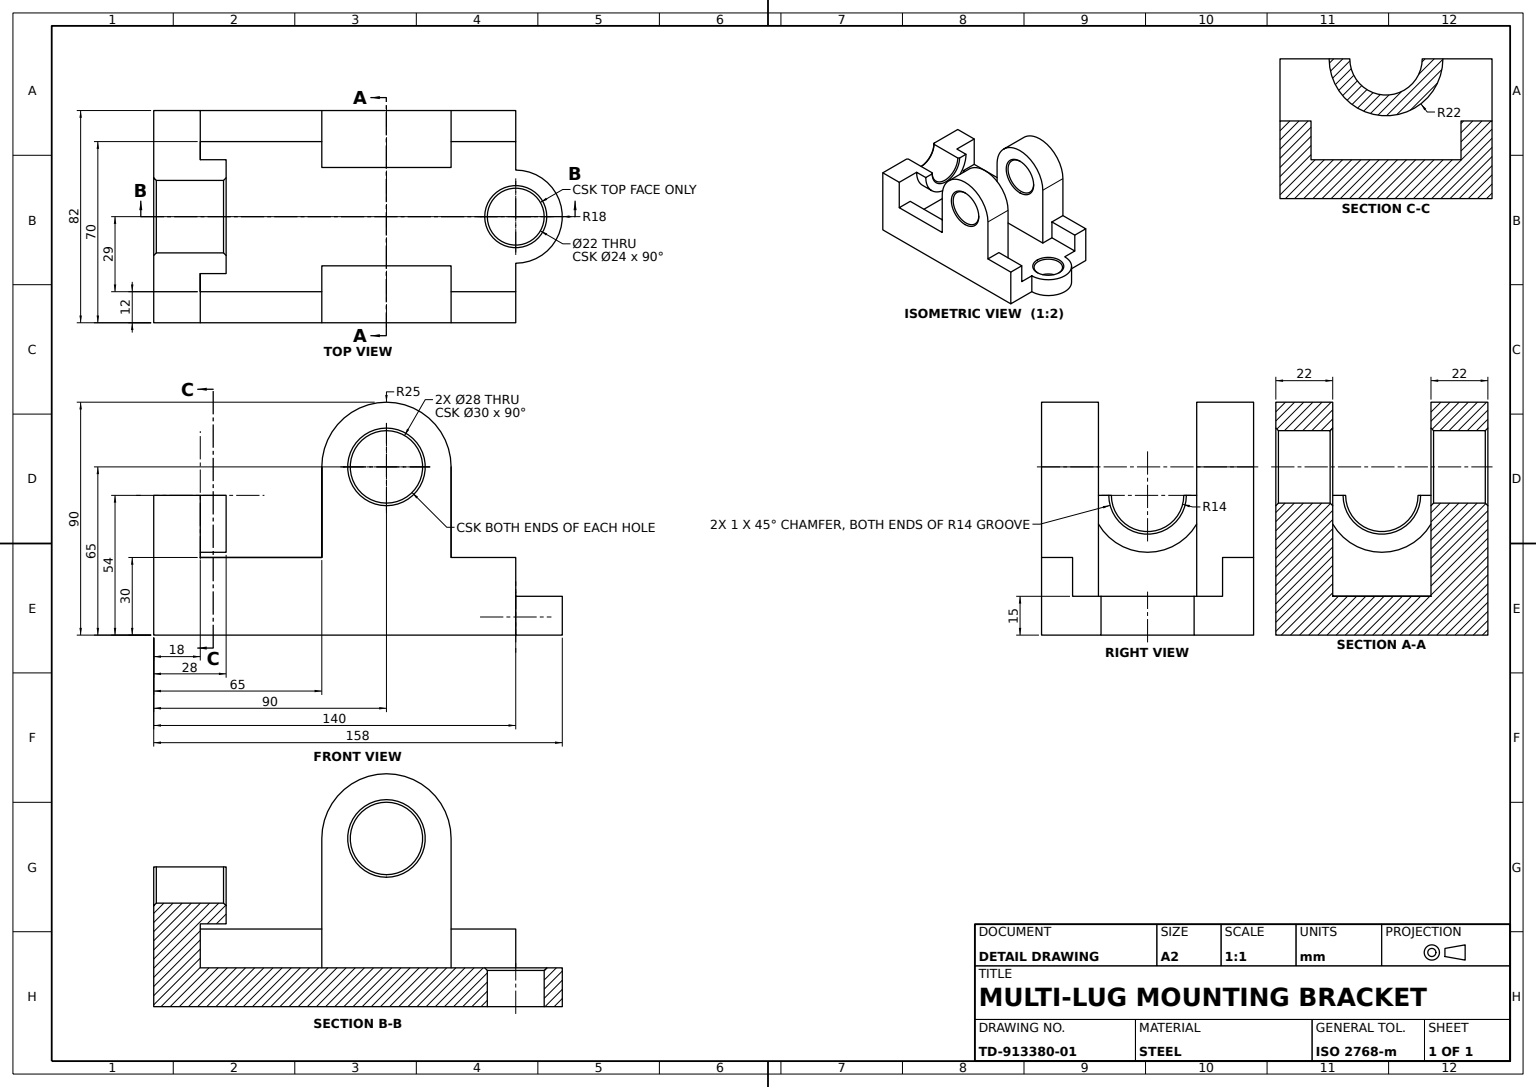
ISO-10303-21;
HEADER;
FILE_DESCRIPTION((''),'2;1');
FILE_NAME('','',(''),(''),'','','');
FILE_SCHEMA(('AUTOMOTIVE_DESIGN'));
ENDSEC;
DATA;
#1=APPLICATION_CONTEXT('');
#2=PRODUCT_CONTEXT('',#1,'mechanical');
#3=PRODUCT('','','',(#2));
#4=PRODUCT_DEFINITION_FORMATION('','',#3);
#5=PRODUCT_DEFINITION_CONTEXT('',#1,'design');
#6=PRODUCT_DEFINITION('','',#4,#5);
#7=PRODUCT_DEFINITION_SHAPE('','',#6);
#8=(LENGTH_UNIT()NAMED_UNIT(*)SI_UNIT(.MILLI.,.METRE.));
#9=(NAMED_UNIT(*)PLANE_ANGLE_UNIT()SI_UNIT($,.RADIAN.));
#10=(NAMED_UNIT(*)SI_UNIT($,.STERADIAN.)SOLID_ANGLE_UNIT());
#11=UNCERTAINTY_MEASURE_WITH_UNIT(LENGTH_MEASURE(0.005),#8,'distance_accuracy_value','');
#12=(GEOMETRIC_REPRESENTATION_CONTEXT(3)GLOBAL_UNCERTAINTY_ASSIGNED_CONTEXT((#11))GLOBAL_UNIT_ASSIGNED_CONTEXT((#8,#9,#10))REPRESENTATION_CONTEXT('',''));
#13=CARTESIAN_POINT('',(-42.,15.,54.));
#14=VERTEX_POINT('',#13);
#15=CARTESIAN_POINT('',(-42.,-15.,54.));
#16=VERTEX_POINT('',#15);
#17=CARTESIAN_POINT('',(-42.,0.,54.));
#18=DIRECTION('',(1.,0.,0.));
#19=DIRECTION('',(0.,0.,-1.));
#20=AXIS2_PLACEMENT_3D('',#17,#18,#19);
#21=CIRCLE('',#20,15.);
#22=EDGE_CURVE('',#14,#16,#21,.F.);
#23=ORIENTED_EDGE('',*,*,#22,.F.);
#24=CARTESIAN_POINT('',(-43.,14.,54.));
#25=VERTEX_POINT('',#24);
#26=CARTESIAN_POINT('',(-57.,0.,54.));
#27=DIRECTION('',(0.707106781,0.707106781,0.));
#28=VECTOR('',#27,1000.);
#29=LINE('',#26,#28);
#30=EDGE_CURVE('',#25,#14,#29,.T.);
#31=ORIENTED_EDGE('',*,*,#30,.F.);
#32=CARTESIAN_POINT('',(-43.,-14.,54.));
#33=VERTEX_POINT('',#32);
#34=CARTESIAN_POINT('',(-43.,0.,54.));
#35=AXIS2_PLACEMENT_3D('',#34,#18,#19);
#36=CIRCLE('',#35,14.);
#37=EDGE_CURVE('',#33,#25,#36,.T.);
#38=ORIENTED_EDGE('',*,*,#37,.F.);
#39=DIRECTION('',(-0.707106781,0.707106781,0.));
#40=VECTOR('',#39,1000.);
#41=LINE('',#26,#40);
#42=EDGE_CURVE('',#16,#33,#41,.T.);
#43=ORIENTED_EDGE('',*,*,#42,.F.);
#44=EDGE_LOOP('',(#23,#31,#38,#43));
#45=FACE_BOUND('',#44,.T.);
#46=CONICAL_SURFACE('',#20,15.,0.785398163);
#47=ADVANCED_FACE('',(#45),#46,.F.);
#48=CARTESIAN_POINT('',(20.,41.,50.));
#49=VERTEX_POINT('',#48);
#50=CARTESIAN_POINT('',(20.,41.,65.));
#51=DIRECTION('',(0.,-1.,0.));
#52=AXIS2_PLACEMENT_3D('',#50,#51,#19);
#53=CIRCLE('',#52,15.);
#54=EDGE_CURVE('',#49,#49,#53,.T.);
#55=ORIENTED_EDGE('',*,*,#54,.T.);
#56=EDGE_LOOP('',(#55));
#57=FACE_BOUND('',#56,.T.);
#58=CARTESIAN_POINT('',(-5.,41.,30.));
#59=VERTEX_POINT('',#58);
#60=CARTESIAN_POINT('',(-52.,41.,30.));
#61=VERTEX_POINT('',#60);
#62=CARTESIAN_POINT('',(70.,41.,30.));
#63=DIRECTION('',(-1.,0.,0.));
#64=VECTOR('',#63,1000.);
#65=LINE('',#62,#64);
#66=EDGE_CURVE('',#59,#61,#65,.T.);
#67=ORIENTED_EDGE('',*,*,#66,.F.);
#68=CARTESIAN_POINT('',(-5.,41.,65.));
#69=VERTEX_POINT('',#68);
#70=VECTOR('',#19,1000.);
#71=LINE('',#68,#70);
#72=EDGE_CURVE('',#69,#59,#71,.T.);
#73=ORIENTED_EDGE('',*,*,#72,.F.);
#74=CARTESIAN_POINT('',(45.,41.,65.));
#75=VERTEX_POINT('',#74);
#76=AXIS2_PLACEMENT_3D('',#50,#51,#18);
#77=CIRCLE('',#76,25.);
#78=EDGE_CURVE('',#75,#69,#77,.T.);
#79=ORIENTED_EDGE('',*,*,#78,.F.);
#80=CARTESIAN_POINT('',(45.,41.,30.));
#81=VERTEX_POINT('',#80);
#82=CARTESIAN_POINT('',(45.,41.,0.));
#83=DIRECTION('',(0.,0.,1.));
#84=VECTOR('',#83,1000.);
#85=LINE('',#82,#84);
#86=EDGE_CURVE('',#81,#75,#85,.T.);
#87=ORIENTED_EDGE('',*,*,#86,.F.);
#88=VERTEX_POINT('',#62);
#89=EDGE_CURVE('',#88,#81,#65,.T.);
#90=ORIENTED_EDGE('',*,*,#89,.F.);
#91=CARTESIAN_POINT('',(70.,41.,0.));
#92=VERTEX_POINT('',#91);
#93=LINE('',#91,#84);
#94=EDGE_CURVE('',#92,#88,#93,.T.);
#95=ORIENTED_EDGE('',*,*,#94,.F.);
#96=CARTESIAN_POINT('',(-70.,41.,0.));
#97=VERTEX_POINT('',#96);
#98=VECTOR('',#18,1000.);
#99=LINE('',#96,#98);
#100=EDGE_CURVE('',#97,#92,#99,.T.);
#101=ORIENTED_EDGE('',*,*,#100,.F.);
#102=CARTESIAN_POINT('',(-70.,41.,54.));
#103=VERTEX_POINT('',#102);
#104=CARTESIAN_POINT('',(-70.,41.,30.));
#105=LINE('',#104,#70);
#106=EDGE_CURVE('',#103,#97,#105,.T.);
#107=ORIENTED_EDGE('',*,*,#106,.F.);
#108=CARTESIAN_POINT('',(-52.,41.,54.));
#109=VERTEX_POINT('',#108);
#110=LINE('',#102,#98);
#111=EDGE_CURVE('',#103,#109,#110,.T.);
#112=ORIENTED_EDGE('',*,*,#111,.T.);
#113=LINE('',#108,#70);
#114=EDGE_CURVE('',#109,#61,#113,.T.);
#115=ORIENTED_EDGE('',*,*,#114,.T.);
#116=EDGE_LOOP('',(#67,#73,#79,#87,#90,#95,#101,#107,#112,#115));
#117=FACE_BOUND('',#116,.T.);
#118=CARTESIAN_POINT('',(0.,41.,0.));
#119=AXIS2_PLACEMENT_3D('',#118,#51,#19);
#120=PLANE('',#119);
#121=ADVANCED_FACE('',(#57,#117),#120,.F.);
#122=CARTESIAN_POINT('',(20.,20.,51.));
#123=VERTEX_POINT('',#122);
#124=CARTESIAN_POINT('',(20.,20.,65.));
#125=AXIS2_PLACEMENT_3D('',#124,#51,#19);
#126=CIRCLE('',#125,14.);
#127=EDGE_CURVE('',#123,#123,#126,.T.);
#128=ORIENTED_EDGE('',*,*,#127,.F.);
#129=EDGE_LOOP('',(#128));
#130=FACE_BOUND('',#129,.T.);
#131=CARTESIAN_POINT('',(20.,19.,50.));
#132=VERTEX_POINT('',#131);
#133=CARTESIAN_POINT('',(20.,19.,65.));
#134=AXIS2_PLACEMENT_3D('',#133,#51,#19);
#135=CIRCLE('',#134,15.);
#136=EDGE_CURVE('',#132,#132,#135,.F.);
#137=ORIENTED_EDGE('',*,*,#136,.F.);
#138=EDGE_LOOP('',(#137));
#139=FACE_BOUND('',#138,.T.);
#140=CONICAL_SURFACE('',#125,14.,0.785398163);
#141=ADVANCED_FACE('',(#130,#139),#140,.F.);
#142=ORIENTED_EDGE('',*,*,#136,.T.);
#143=EDGE_LOOP('',(#142));
#144=FACE_BOUND('',#143,.T.);
#145=CARTESIAN_POINT('',(45.,19.,65.));
#146=VERTEX_POINT('',#145);
#147=CARTESIAN_POINT('',(-5.,19.,65.));
#148=VERTEX_POINT('',#147);
#149=AXIS2_PLACEMENT_3D('',#133,#51,#18);
#150=CIRCLE('',#149,25.);
#151=EDGE_CURVE('',#146,#148,#150,.T.);
#152=ORIENTED_EDGE('',*,*,#151,.T.);
#153=CARTESIAN_POINT('',(-5.,19.,15.));
#154=VERTEX_POINT('',#153);
#155=LINE('',#147,#70);
#156=EDGE_CURVE('',#148,#154,#155,.T.);
#157=ORIENTED_EDGE('',*,*,#156,.T.);
#158=CARTESIAN_POINT('',(45.,19.,15.));
#159=VERTEX_POINT('',#158);
#160=CARTESIAN_POINT('',(0.,19.,15.));
#161=LINE('',#160,#64);
#162=EDGE_CURVE('',#159,#154,#161,.T.);
#163=ORIENTED_EDGE('',*,*,#162,.F.);
#164=CARTESIAN_POINT('',(45.,19.,0.));
#165=LINE('',#164,#84);
#166=EDGE_CURVE('',#159,#146,#165,.T.);
#167=ORIENTED_EDGE('',*,*,#166,.T.);
#168=EDGE_LOOP('',(#152,#157,#163,#167));
#169=FACE_BOUND('',#168,.T.);
#170=PLANE('',#134);
#171=ADVANCED_FACE('',(#144,#169),#170,.T.);
#172=CARTESIAN_POINT('',(-5.,-29.,15.));
#173=VERTEX_POINT('',#172);
#174=CARTESIAN_POINT('',(-5.,-29.,30.));
#175=VERTEX_POINT('',#174);
#176=CARTESIAN_POINT('',(-5.,-29.,47.));
#177=LINE('',#176,#84);
#178=EDGE_CURVE('',#173,#175,#177,.T.);
#179=ORIENTED_EDGE('',*,*,#178,.T.);
#180=CARTESIAN_POINT('',(-5.,-41.,30.));
#181=VERTEX_POINT('',#180);
#182=DIRECTION('',(0.,1.,0.));
#183=VECTOR('',#182,1000.);
#184=LINE('',#58,#183);
#185=EDGE_CURVE('',#181,#175,#184,.T.);
#186=ORIENTED_EDGE('',*,*,#185,.F.);
#187=CARTESIAN_POINT('',(-5.,-41.,65.));
#188=VERTEX_POINT('',#187);
#189=LINE('',#187,#70);
#190=EDGE_CURVE('',#188,#181,#189,.T.);
#191=ORIENTED_EDGE('',*,*,#190,.F.);
#192=CARTESIAN_POINT('',(-5.,-19.,65.));
#193=VERTEX_POINT('',#192);
#194=LINE('',#187,#183);
#195=EDGE_CURVE('',#188,#193,#194,.T.);
#196=ORIENTED_EDGE('',*,*,#195,.T.);
#197=CARTESIAN_POINT('',(-5.,-19.,15.));
#198=VERTEX_POINT('',#197);
#199=LINE('',#192,#70);
#200=EDGE_CURVE('',#193,#198,#199,.T.);
#201=ORIENTED_EDGE('',*,*,#200,.T.);
#202=CARTESIAN_POINT('',(-5.,0.,15.));
#203=VECTOR('',#51,1000.);
#204=LINE('',#202,#203);
#205=EDGE_CURVE('',#198,#173,#204,.T.);
#206=ORIENTED_EDGE('',*,*,#205,.T.);
#207=EDGE_LOOP('',(#179,#186,#191,#196,#201,#206));
#208=FACE_BOUND('',#207,.T.);
#209=AXIS2_PLACEMENT_3D('',#187,#18,#19);
#210=PLANE('',#209);
#211=ADVANCED_FACE('',(#208),#210,.F.);
#212=CARTESIAN_POINT('',(70.,29.,15.));
#213=VERTEX_POINT('',#212);
#214=CARTESIAN_POINT('',(70.,29.,30.));
#215=VERTEX_POINT('',#214);
#216=CARTESIAN_POINT('',(70.,29.,47.));
#217=LINE('',#216,#70);
#218=EDGE_CURVE('',#213,#215,#217,.F.);
#219=ORIENTED_EDGE('',*,*,#218,.T.);
#220=CARTESIAN_POINT('',(45.,29.,30.));
#221=VERTEX_POINT('',#220);
#222=LINE('',#214,#64);
#223=EDGE_CURVE('',#215,#221,#222,.T.);
#224=ORIENTED_EDGE('',*,*,#223,.T.);
#225=CARTESIAN_POINT('',(45.,29.,15.));
#226=VERTEX_POINT('',#225);
#227=CARTESIAN_POINT('',(45.,29.,47.));
#228=LINE('',#227,#70);
#229=EDGE_CURVE('',#221,#226,#228,.T.);
#230=ORIENTED_EDGE('',*,*,#229,.T.);
#231=CARTESIAN_POINT('',(-52.,29.,15.));
#232=LINE('',#231,#98);
#233=EDGE_CURVE('',#213,#226,#232,.F.);
#234=ORIENTED_EDGE('',*,*,#233,.F.);
#235=EDGE_LOOP('',(#219,#224,#230,#234));
#236=FACE_BOUND('',#235,.T.);
#237=CARTESIAN_POINT('',(-52.,29.,47.));
#238=AXIS2_PLACEMENT_3D('',#237,#182,#83);
#239=PLANE('',#238);
#240=ADVANCED_FACE('',(#236),#239,.F.);
#241=CARTESIAN_POINT('',(20.,-20.,51.));
#242=VERTEX_POINT('',#241);
#243=CARTESIAN_POINT('',(20.,-20.,65.));
#244=AXIS2_PLACEMENT_3D('',#243,#51,#19);
#245=CIRCLE('',#244,14.);
#246=EDGE_CURVE('',#242,#242,#245,.F.);
#247=ORIENTED_EDGE('',*,*,#246,.F.);
#248=EDGE_LOOP('',(#247));
#249=FACE_BOUND('',#248,.T.);
#250=CARTESIAN_POINT('',(20.,-19.,50.));
#251=VERTEX_POINT('',#250);
#252=CARTESIAN_POINT('',(20.,-19.,65.));
#253=AXIS2_PLACEMENT_3D('',#252,#51,#19);
#254=CIRCLE('',#253,15.);
#255=EDGE_CURVE('',#251,#251,#254,.T.);
#256=ORIENTED_EDGE('',*,*,#255,.F.);
#257=EDGE_LOOP('',(#256));
#258=FACE_BOUND('',#257,.T.);
#259=AXIS2_PLACEMENT_3D('',#252,#182,#83);
#260=CONICAL_SURFACE('',#259,15.,0.785398163);
#261=ADVANCED_FACE('',(#249,#258),#260,.F.);
#262=CARTESIAN_POINT('',(-5.,29.,30.));
#263=VERTEX_POINT('',#262);
#264=CARTESIAN_POINT('',(-52.,29.,30.));
#265=VERTEX_POINT('',#264);
#266=EDGE_CURVE('',#263,#265,#222,.T.);
#267=ORIENTED_EDGE('',*,*,#266,.T.);
#268=VERTEX_POINT('',#231);
#269=LINE('',#237,#70);
#270=EDGE_CURVE('',#268,#265,#269,.F.);
#271=ORIENTED_EDGE('',*,*,#270,.F.);
#272=CARTESIAN_POINT('',(-5.,29.,15.));
#273=VERTEX_POINT('',#272);
#274=EDGE_CURVE('',#273,#268,#232,.F.);
#275=ORIENTED_EDGE('',*,*,#274,.F.);
#276=CARTESIAN_POINT('',(-5.,29.,47.));
#277=LINE('',#276,#84);
#278=EDGE_CURVE('',#273,#263,#277,.T.);
#279=ORIENTED_EDGE('',*,*,#278,.T.);
#280=EDGE_LOOP('',(#267,#271,#275,#279));
#281=FACE_BOUND('',#280,.T.);
#282=ADVANCED_FACE('',(#281),#239,.F.);
#283=CARTESIAN_POINT('',(45.,-29.,30.));
#284=VERTEX_POINT('',#283);
#285=CARTESIAN_POINT('',(45.,-29.,15.));
#286=VERTEX_POINT('',#285);
#287=CARTESIAN_POINT('',(45.,-29.,47.));
#288=LINE('',#287,#70);
#289=EDGE_CURVE('',#284,#286,#288,.T.);
#290=ORIENTED_EDGE('',*,*,#289,.F.);
#291=CARTESIAN_POINT('',(70.,-29.,30.));
#292=VERTEX_POINT('',#291);
#293=LINE('',#291,#98);
#294=EDGE_CURVE('',#284,#292,#293,.T.);
#295=ORIENTED_EDGE('',*,*,#294,.T.);
#296=CARTESIAN_POINT('',(70.,-29.,15.));
#297=VERTEX_POINT('',#296);
#298=CARTESIAN_POINT('',(70.,-29.,47.));
#299=LINE('',#298,#70);
#300=EDGE_CURVE('',#297,#292,#299,.F.);
#301=ORIENTED_EDGE('',*,*,#300,.F.);
#302=LINE('',#296,#64);
#303=EDGE_CURVE('',#286,#297,#302,.F.);
#304=ORIENTED_EDGE('',*,*,#303,.F.);
#305=EDGE_LOOP('',(#290,#295,#301,#304));
#306=FACE_BOUND('',#305,.T.);
#307=AXIS2_PLACEMENT_3D('',#298,#51,#19);
#308=PLANE('',#307);
#309=ADVANCED_FACE('',(#306),#308,.F.);
#310=ORIENTED_EDGE('',*,*,#246,.T.);
#311=EDGE_LOOP('',(#310));
#312=FACE_BOUND('',#311,.T.);
#313=CARTESIAN_POINT('',(20.,-40.,51.));
#314=VERTEX_POINT('',#313);
#315=CARTESIAN_POINT('',(20.,-40.,65.));
#316=AXIS2_PLACEMENT_3D('',#315,#51,#19);
#317=CIRCLE('',#316,14.);
#318=EDGE_CURVE('',#314,#314,#317,.T.);
#319=ORIENTED_EDGE('',*,*,#318,.T.);
#320=EDGE_LOOP('',(#319));
#321=FACE_BOUND('',#320,.T.);
#322=CARTESIAN_POINT('',(20.,-41.,65.));
#323=AXIS2_PLACEMENT_3D('',#322,#182,#83);
#324=CYLINDRICAL_SURFACE('',#323,14.);
#325=ADVANCED_FACE('',(#312,#321),#324,.F.);
#326=CARTESIAN_POINT('',(-70.,-41.,54.));
#327=VERTEX_POINT('',#326);
#328=CARTESIAN_POINT('',(-70.,-15.,54.));
#329=VERTEX_POINT('',#328);
#330=LINE('',#326,#183);
#331=EDGE_CURVE('',#327,#329,#330,.T.);
#332=ORIENTED_EDGE('',*,*,#331,.T.);
#333=CARTESIAN_POINT('',(-70.,15.,54.));
#334=VERTEX_POINT('',#333);
#335=CARTESIAN_POINT('',(-70.,0.,54.));
#336=AXIS2_PLACEMENT_3D('',#335,#63,#83);
#337=CIRCLE('',#336,15.);
#338=EDGE_CURVE('',#329,#334,#337,.F.);
#339=ORIENTED_EDGE('',*,*,#338,.T.);
#340=EDGE_CURVE('',#334,#103,#330,.T.);
#341=ORIENTED_EDGE('',*,*,#340,.T.);
#342=ORIENTED_EDGE('',*,*,#106,.T.);
#343=CARTESIAN_POINT('',(-70.,-41.,0.));
#344=VERTEX_POINT('',#343);
#345=LINE('',#96,#203);
#346=EDGE_CURVE('',#97,#344,#345,.T.);
#347=ORIENTED_EDGE('',*,*,#346,.T.);
#348=CARTESIAN_POINT('',(-70.,-41.,30.));
#349=LINE('',#348,#70);
#350=EDGE_CURVE('',#327,#344,#349,.T.);
#351=ORIENTED_EDGE('',*,*,#350,.F.);
#352=EDGE_LOOP('',(#332,#339,#341,#342,#347,#351));
#353=FACE_BOUND('',#352,.T.);
#354=AXIS2_PLACEMENT_3D('',#104,#63,#83);
#355=PLANE('',#354);
#356=ADVANCED_FACE('',(#353),#355,.T.);
#357=ORIENTED_EDGE('',*,*,#78,.T.);
#358=LINE('',#68,#203);
#359=EDGE_CURVE('',#69,#148,#358,.T.);
#360=ORIENTED_EDGE('',*,*,#359,.T.);
#361=ORIENTED_EDGE('',*,*,#151,.F.);
#362=LINE('',#74,#203);
#363=EDGE_CURVE('',#75,#146,#362,.T.);
#364=ORIENTED_EDGE('',*,*,#363,.F.);
#365=EDGE_LOOP('',(#357,#360,#361,#364));
#366=FACE_BOUND('',#365,.T.);
#367=CYLINDRICAL_SURFACE('',#52,25.);
#368=ADVANCED_FACE('',(#366),#367,.T.);
#369=ORIENTED_EDGE('',*,*,#66,.T.);
#370=LINE('',#60,#183);
#371=EDGE_CURVE('',#265,#61,#370,.T.);
#372=ORIENTED_EDGE('',*,*,#371,.F.);
#373=ORIENTED_EDGE('',*,*,#266,.F.);
#374=LINE('',#58,#203);
#375=EDGE_CURVE('',#59,#263,#374,.T.);
#376=ORIENTED_EDGE('',*,*,#375,.F.);
#377=EDGE_LOOP('',(#369,#372,#373,#376));
#378=FACE_BOUND('',#377,.T.);
#379=AXIS2_PLACEMENT_3D('',#62,#83,#18);
#380=PLANE('',#379);
#381=ADVANCED_FACE('',(#378),#380,.T.);
#382=CARTESIAN_POINT('',(58.,0.,15.));
#383=VERTEX_POINT('',#382);
#384=CARTESIAN_POINT('',(70.,0.,15.));
#385=AXIS2_PLACEMENT_3D('',#384,#19,#63);
#386=CIRCLE('',#385,12.);
#387=EDGE_CURVE('',#383,#383,#386,.T.);
#388=ORIENTED_EDGE('',*,*,#387,.F.);
#389=EDGE_LOOP('',(#388));
#390=FACE_BOUND('',#389,.T.);
#391=CARTESIAN_POINT('',(59.,0.,14.));
#392=VERTEX_POINT('',#391);
#393=CARTESIAN_POINT('',(70.,0.,14.));
#394=AXIS2_PLACEMENT_3D('',#393,#19,#63);
#395=CIRCLE('',#394,11.);
#396=EDGE_CURVE('',#392,#392,#395,.F.);
#397=ORIENTED_EDGE('',*,*,#396,.F.);
#398=EDGE_LOOP('',(#397));
#399=FACE_BOUND('',#398,.T.);
#400=AXIS2_PLACEMENT_3D('',#384,#83,#18);
#401=CONICAL_SURFACE('',#400,12.,0.785398163);
#402=ADVANCED_FACE('',(#390,#399),#401,.F.);
#403=CARTESIAN_POINT('',(20.,-41.,50.));
#404=VERTEX_POINT('',#403);
#405=AXIS2_PLACEMENT_3D('',#322,#51,#19);
#406=CIRCLE('',#405,15.);
#407=EDGE_CURVE('',#404,#404,#406,.F.);
#408=ORIENTED_EDGE('',*,*,#407,.F.);
#409=EDGE_LOOP('',(#408));
#410=FACE_BOUND('',#409,.T.);
#411=ORIENTED_EDGE('',*,*,#318,.F.);
#412=EDGE_LOOP('',(#411));
#413=FACE_BOUND('',#412,.T.);
#414=CONICAL_SURFACE('',#405,15.,0.785398163);
#415=ADVANCED_FACE('',(#410,#413),#414,.F.);
#416=CARTESIAN_POINT('',(45.,-19.,65.));
#417=VERTEX_POINT('',#416);
#418=AXIS2_PLACEMENT_3D('',#252,#51,#18);
#419=CIRCLE('',#418,25.);
#420=EDGE_CURVE('',#417,#193,#419,.T.);
#421=ORIENTED_EDGE('',*,*,#420,.T.);
#422=ORIENTED_EDGE('',*,*,#195,.F.);
#423=CARTESIAN_POINT('',(45.,-41.,65.));
#424=VERTEX_POINT('',#423);
#425=AXIS2_PLACEMENT_3D('',#322,#51,#18);
#426=CIRCLE('',#425,25.);
#427=EDGE_CURVE('',#424,#188,#426,.T.);
#428=ORIENTED_EDGE('',*,*,#427,.F.);
#429=LINE('',#423,#183);
#430=EDGE_CURVE('',#424,#417,#429,.T.);
#431=ORIENTED_EDGE('',*,*,#430,.T.);
#432=EDGE_LOOP('',(#421,#422,#428,#431));
#433=FACE_BOUND('',#432,.T.);
#434=CYLINDRICAL_SURFACE('',#323,25.);
#435=ADVANCED_FACE('',(#433),#434,.T.);
#436=CARTESIAN_POINT('',(70.,18.,0.));
#437=VERTEX_POINT('',#436);
#438=CARTESIAN_POINT('',(70.,18.,15.));
#439=VERTEX_POINT('',#438);
#440=LINE('',#438,#70);
#441=EDGE_CURVE('',#437,#439,#440,.F.);
#442=ORIENTED_EDGE('',*,*,#441,.T.);
#443=CARTESIAN_POINT('',(70.,-18.,15.));
#444=VERTEX_POINT('',#443);
#445=AXIS2_PLACEMENT_3D('',#384,#19,#18);
#446=CIRCLE('',#445,18.);
#447=EDGE_CURVE('',#439,#444,#446,.T.);
#448=ORIENTED_EDGE('',*,*,#447,.T.);
#449=CARTESIAN_POINT('',(70.,-18.,0.));
#450=VERTEX_POINT('',#449);
#451=LINE('',#443,#70);
#452=EDGE_CURVE('',#444,#450,#451,.T.);
#453=ORIENTED_EDGE('',*,*,#452,.T.);
#454=CARTESIAN_POINT('',(70.,0.,0.));
#455=AXIS2_PLACEMENT_3D('',#454,#19,#18);
#456=CIRCLE('',#455,18.);
#457=EDGE_CURVE('',#437,#450,#456,.T.);
#458=ORIENTED_EDGE('',*,*,#457,.F.);
#459=EDGE_LOOP('',(#442,#448,#453,#458));
#460=FACE_BOUND('',#459,.T.);
#461=CYLINDRICAL_SURFACE('',#385,18.);
#462=ADVANCED_FACE('',(#460),#461,.T.);
#463=LINE('',#80,#183);
#464=EDGE_CURVE('',#221,#81,#463,.T.);
#465=ORIENTED_EDGE('',*,*,#464,.F.);
#466=ORIENTED_EDGE('',*,*,#223,.F.);
#467=LINE('',#62,#203);
#468=EDGE_CURVE('',#88,#215,#467,.T.);
#469=ORIENTED_EDGE('',*,*,#468,.F.);
#470=ORIENTED_EDGE('',*,*,#89,.T.);
#471=EDGE_LOOP('',(#465,#466,#469,#470));
#472=FACE_BOUND('',#471,.T.);
#473=ADVANCED_FACE('',(#472),#380,.T.);
#474=ORIENTED_EDGE('',*,*,#274,.T.);
#475=CARTESIAN_POINT('',(-52.,-29.,15.));
#476=VERTEX_POINT('',#475);
#477=LINE('',#475,#183);
#478=EDGE_CURVE('',#268,#476,#477,.F.);
#479=ORIENTED_EDGE('',*,*,#478,.T.);
#480=EDGE_CURVE('',#476,#173,#302,.F.);
#481=ORIENTED_EDGE('',*,*,#480,.T.);
#482=ORIENTED_EDGE('',*,*,#205,.F.);
#483=CARTESIAN_POINT('',(45.,-19.,15.));
#484=VERTEX_POINT('',#483);
#485=CARTESIAN_POINT('',(0.,-19.,15.));
#486=LINE('',#485,#64);
#487=EDGE_CURVE('',#484,#198,#486,.T.);
#488=ORIENTED_EDGE('',*,*,#487,.F.);
#489=CARTESIAN_POINT('',(45.,0.,15.));
#490=LINE('',#489,#183);
#491=EDGE_CURVE('',#286,#484,#490,.T.);
#492=ORIENTED_EDGE('',*,*,#491,.F.);
#493=ORIENTED_EDGE('',*,*,#303,.T.);
#494=LINE('',#212,#203);
#495=EDGE_CURVE('',#444,#297,#494,.T.);
#496=ORIENTED_EDGE('',*,*,#495,.F.);
#497=ORIENTED_EDGE('',*,*,#447,.F.);
#498=EDGE_CURVE('',#213,#439,#494,.T.);
#499=ORIENTED_EDGE('',*,*,#498,.F.);
#500=ORIENTED_EDGE('',*,*,#233,.T.);
#501=LINE('',#489,#203);
#502=EDGE_CURVE('',#226,#159,#501,.T.);
#503=ORIENTED_EDGE('',*,*,#502,.T.);
#504=ORIENTED_EDGE('',*,*,#162,.T.);
#505=LINE('',#202,#183);
#506=EDGE_CURVE('',#154,#273,#505,.T.);
#507=ORIENTED_EDGE('',*,*,#506,.T.);
#508=EDGE_LOOP('',(#474,#479,#481,#482,#488,#492,#493,#496,#497,#499,#500,#503,#504,#507));
#509=FACE_BOUND('',#508,.T.);
#510=ORIENTED_EDGE('',*,*,#387,.T.);
#511=EDGE_LOOP('',(#510));
#512=FACE_BOUND('',#511,.T.);
#513=CARTESIAN_POINT('',(0.,0.,15.));
#514=AXIS2_PLACEMENT_3D('',#513,#19,#63);
#515=PLANE('',#514);
#516=ADVANCED_FACE('',(#509,#512),#515,.F.);
#517=CARTESIAN_POINT('',(20.,40.,51.));
#518=VERTEX_POINT('',#517);
#519=CARTESIAN_POINT('',(20.,40.,65.));
#520=AXIS2_PLACEMENT_3D('',#519,#51,#19);
#521=CIRCLE('',#520,14.);
#522=EDGE_CURVE('',#518,#518,#521,.F.);
#523=ORIENTED_EDGE('',*,*,#522,.T.);
#524=EDGE_LOOP('',(#523));
#525=FACE_BOUND('',#524,.T.);
#526=ORIENTED_EDGE('',*,*,#127,.T.);
#527=EDGE_LOOP('',(#526));
#528=FACE_BOUND('',#527,.T.);
#529=ADVANCED_FACE('',(#525,#528),#324,.F.);
#530=ORIENTED_EDGE('',*,*,#371,.T.);
#531=ORIENTED_EDGE('',*,*,#114,.F.);
#532=CARTESIAN_POINT('',(-52.,22.,54.));
#533=VERTEX_POINT('',#532);
#534=LINE('',#108,#203);
#535=EDGE_CURVE('',#109,#533,#534,.T.);
#536=ORIENTED_EDGE('',*,*,#535,.T.);
#537=CARTESIAN_POINT('',(-52.,-22.,54.));
#538=VERTEX_POINT('',#537);
#539=CARTESIAN_POINT('',(-52.,0.,54.));
#540=AXIS2_PLACEMENT_3D('',#539,#63,#51);
#541=CIRCLE('',#540,22.);
#542=EDGE_CURVE('',#533,#538,#541,.T.);
#543=ORIENTED_EDGE('',*,*,#542,.T.);
#544=CARTESIAN_POINT('',(-52.,-41.,54.));
#545=VERTEX_POINT('',#544);
#546=EDGE_CURVE('',#538,#545,#534,.T.);
#547=ORIENTED_EDGE('',*,*,#546,.T.);
#548=CARTESIAN_POINT('',(-52.,-41.,30.));
#549=VERTEX_POINT('',#548);
#550=LINE('',#544,#70);
#551=EDGE_CURVE('',#545,#549,#550,.T.);
#552=ORIENTED_EDGE('',*,*,#551,.T.);
#553=CARTESIAN_POINT('',(-52.,-29.,30.));
#554=VERTEX_POINT('',#553);
#555=EDGE_CURVE('',#549,#554,#370,.T.);
#556=ORIENTED_EDGE('',*,*,#555,.T.);
#557=CARTESIAN_POINT('',(-52.,-29.,47.));
#558=LINE('',#557,#70);
#559=EDGE_CURVE('',#476,#554,#558,.F.);
#560=ORIENTED_EDGE('',*,*,#559,.F.);
#561=ORIENTED_EDGE('',*,*,#478,.F.);
#562=ORIENTED_EDGE('',*,*,#270,.T.);
#563=EDGE_LOOP('',(#530,#531,#536,#543,#547,#552,#556,#560,#561,#562));
#564=FACE_BOUND('',#563,.T.);
#565=AXIS2_PLACEMENT_3D('',#557,#63,#51);
#566=PLANE('',#565);
#567=ADVANCED_FACE('',(#564),#566,.F.);
#568=ORIENTED_EDGE('',*,*,#359,.F.);
#569=ORIENTED_EDGE('',*,*,#72,.T.);
#570=ORIENTED_EDGE('',*,*,#375,.T.);
#571=ORIENTED_EDGE('',*,*,#278,.F.);
#572=ORIENTED_EDGE('',*,*,#506,.F.);
#573=ORIENTED_EDGE('',*,*,#156,.F.);
#574=EDGE_LOOP('',(#568,#569,#570,#571,#572,#573));
#575=FACE_BOUND('',#574,.T.);
#576=AXIS2_PLACEMENT_3D('',#68,#63,#83);
#577=PLANE('',#576);
#578=ADVANCED_FACE('',(#575),#577,.T.);
#579=ORIENTED_EDGE('',*,*,#166,.F.);
#580=ORIENTED_EDGE('',*,*,#502,.F.);
#581=ORIENTED_EDGE('',*,*,#229,.F.);
#582=ORIENTED_EDGE('',*,*,#464,.T.);
#583=ORIENTED_EDGE('',*,*,#86,.T.);
#584=ORIENTED_EDGE('',*,*,#363,.T.);
#585=EDGE_LOOP('',(#579,#580,#581,#582,#583,#584));
#586=FACE_BOUND('',#585,.T.);
#587=AXIS2_PLACEMENT_3D('',#82,#18,#19);
#588=PLANE('',#587);
#589=ADVANCED_FACE('',(#586),#588,.T.);
#590=CARTESIAN_POINT('',(-69.,14.,54.));
#591=VERTEX_POINT('',#590);
#592=CARTESIAN_POINT('',(-55.,0.,54.));
#593=DIRECTION('',(0.707106781,-0.707106781,0.));
#594=VECTOR('',#593,1000.);
#595=LINE('',#592,#594);
#596=EDGE_CURVE('',#334,#591,#595,.T.);
#597=ORIENTED_EDGE('',*,*,#596,.F.);
#598=ORIENTED_EDGE('',*,*,#338,.F.);
#599=CARTESIAN_POINT('',(-69.,-14.,54.));
#600=VERTEX_POINT('',#599);
#601=DIRECTION('',(-0.707106781,-0.707106781,0.));
#602=VECTOR('',#601,1000.);
#603=LINE('',#592,#602);
#604=EDGE_CURVE('',#600,#329,#603,.T.);
#605=ORIENTED_EDGE('',*,*,#604,.F.);
#606=CARTESIAN_POINT('',(-69.,0.,54.));
#607=AXIS2_PLACEMENT_3D('',#606,#63,#83);
#608=CIRCLE('',#607,14.);
#609=EDGE_CURVE('',#591,#600,#608,.T.);
#610=ORIENTED_EDGE('',*,*,#609,.F.);
#611=EDGE_LOOP('',(#597,#598,#605,#610));
#612=FACE_BOUND('',#611,.T.);
#613=CONICAL_SURFACE('',#607,14.,0.785398163);
#614=ADVANCED_FACE('',(#612),#613,.F.);
#615=ORIENTED_EDGE('',*,*,#542,.F.);
#616=CARTESIAN_POINT('',(-42.,22.,54.));
#617=VERTEX_POINT('',#616);
#618=CARTESIAN_POINT('',(-70.,22.,54.));
#619=LINE('',#618,#98);
#620=EDGE_CURVE('',#617,#533,#619,.F.);
#621=ORIENTED_EDGE('',*,*,#620,.F.);
#622=CARTESIAN_POINT('',(-42.,-22.,54.));
#623=VERTEX_POINT('',#622);
#624=AXIS2_PLACEMENT_3D('',#17,#18,#182);
#625=CIRCLE('',#624,22.);
#626=EDGE_CURVE('',#623,#617,#625,.T.);
#627=ORIENTED_EDGE('',*,*,#626,.F.);
#628=CARTESIAN_POINT('',(-70.,-22.,54.));
#629=LINE('',#628,#98);
#630=EDGE_CURVE('',#538,#623,#629,.T.);
#631=ORIENTED_EDGE('',*,*,#630,.F.);
#632=EDGE_LOOP('',(#615,#621,#627,#631));
#633=FACE_BOUND('',#632,.T.);
#634=AXIS2_PLACEMENT_3D('',#335,#18,#19);
#635=CYLINDRICAL_SURFACE('',#634,22.);
#636=ADVANCED_FACE('',(#633),#635,.T.);
#637=CARTESIAN_POINT('',(59.,0.,0.));
#638=VERTEX_POINT('',#637);
#639=AXIS2_PLACEMENT_3D('',#454,#19,#63);
#640=CIRCLE('',#639,11.);
#641=EDGE_CURVE('',#638,#638,#640,.T.);
#642=ORIENTED_EDGE('',*,*,#641,.F.);
#643=EDGE_LOOP('',(#642));
#644=FACE_BOUND('',#643,.T.);
#645=CARTESIAN_POINT('',(70.,-41.,0.));
#646=VERTEX_POINT('',#645);
#647=LINE('',#343,#98);
#648=EDGE_CURVE('',#344,#646,#647,.T.);
#649=ORIENTED_EDGE('',*,*,#648,.F.);
#650=ORIENTED_EDGE('',*,*,#346,.F.);
#651=ORIENTED_EDGE('',*,*,#100,.T.);
#652=LINE('',#91,#203);
#653=EDGE_CURVE('',#92,#437,#652,.T.);
#654=ORIENTED_EDGE('',*,*,#653,.T.);
#655=ORIENTED_EDGE('',*,*,#457,.T.);
#656=EDGE_CURVE('',#450,#646,#652,.T.);
#657=ORIENTED_EDGE('',*,*,#656,.T.);
#658=EDGE_LOOP('',(#649,#650,#651,#654,#655,#657));
#659=FACE_BOUND('',#658,.T.);
#660=AXIS2_PLACEMENT_3D('',#96,#19,#63);
#661=PLANE('',#660);
#662=ADVANCED_FACE('',(#644,#659),#661,.T.);
#663=ORIENTED_EDGE('',*,*,#255,.T.);
#664=EDGE_LOOP('',(#663));
#665=FACE_BOUND('',#664,.T.);
#666=ORIENTED_EDGE('',*,*,#420,.F.);
#667=CARTESIAN_POINT('',(45.,-19.,0.));
#668=LINE('',#667,#84);
#669=EDGE_CURVE('',#484,#417,#668,.T.);
#670=ORIENTED_EDGE('',*,*,#669,.F.);
#671=ORIENTED_EDGE('',*,*,#487,.T.);
#672=ORIENTED_EDGE('',*,*,#200,.F.);
#673=EDGE_LOOP('',(#666,#670,#671,#672));
#674=FACE_BOUND('',#673,.T.);
#675=PLANE('',#253);
#676=ADVANCED_FACE('',(#665,#674),#675,.F.);
#677=LINE('',#17,#183);
#678=EDGE_CURVE('',#623,#16,#677,.T.);
#679=ORIENTED_EDGE('',*,*,#678,.T.);
#680=ORIENTED_EDGE('',*,*,#42,.T.);
#681=CARTESIAN_POINT('',(-42.,-14.,54.));
#682=LINE('',#681,#64);
#683=EDGE_CURVE('',#600,#33,#682,.F.);
#684=ORIENTED_EDGE('',*,*,#683,.F.);
#685=ORIENTED_EDGE('',*,*,#604,.T.);
#686=ORIENTED_EDGE('',*,*,#331,.F.);
#687=LINE('',#544,#64);
#688=EDGE_CURVE('',#545,#327,#687,.T.);
#689=ORIENTED_EDGE('',*,*,#688,.F.);
#690=ORIENTED_EDGE('',*,*,#546,.F.);
#691=ORIENTED_EDGE('',*,*,#630,.T.);
#692=EDGE_LOOP('',(#679,#680,#684,#685,#686,#689,#690,#691));
#693=FACE_BOUND('',#692,.T.);
#694=CARTESIAN_POINT('',(0.,0.,54.));
#695=AXIS2_PLACEMENT_3D('',#694,#19,#63);
#696=PLANE('',#695);
#697=ADVANCED_FACE('',(#693),#696,.F.);
#698=CARTESIAN_POINT('',(45.,-41.,30.));
#699=VERTEX_POINT('',#698);
#700=CARTESIAN_POINT('',(45.,-41.,0.));
#701=LINE('',#700,#84);
#702=EDGE_CURVE('',#699,#424,#701,.T.);
#703=ORIENTED_EDGE('',*,*,#702,.T.);
#704=ORIENTED_EDGE('',*,*,#427,.T.);
#705=ORIENTED_EDGE('',*,*,#190,.T.);
#706=CARTESIAN_POINT('',(70.,-41.,30.));
#707=LINE('',#706,#64);
#708=EDGE_CURVE('',#181,#549,#707,.T.);
#709=ORIENTED_EDGE('',*,*,#708,.T.);
#710=ORIENTED_EDGE('',*,*,#551,.F.);
#711=ORIENTED_EDGE('',*,*,#688,.T.);
#712=ORIENTED_EDGE('',*,*,#350,.T.);
#713=ORIENTED_EDGE('',*,*,#648,.T.);
#714=VERTEX_POINT('',#706);
#715=LINE('',#645,#84);
#716=EDGE_CURVE('',#646,#714,#715,.T.);
#717=ORIENTED_EDGE('',*,*,#716,.T.);
#718=EDGE_CURVE('',#714,#699,#707,.T.);
#719=ORIENTED_EDGE('',*,*,#718,.T.);
#720=EDGE_LOOP('',(#703,#704,#705,#709,#710,#711,#712,#713,#717,#719));
#721=FACE_BOUND('',#720,.T.);
#722=ORIENTED_EDGE('',*,*,#407,.T.);
#723=EDGE_LOOP('',(#722));
#724=FACE_BOUND('',#723,.T.);
#725=CARTESIAN_POINT('',(0.,-41.,0.));
#726=AXIS2_PLACEMENT_3D('',#725,#51,#19);
#727=PLANE('',#726);
#728=ADVANCED_FACE('',(#721,#724),#727,.T.);
#729=ORIENTED_EDGE('',*,*,#111,.F.);
#730=ORIENTED_EDGE('',*,*,#340,.F.);
#731=ORIENTED_EDGE('',*,*,#596,.T.);
#732=CARTESIAN_POINT('',(-42.,14.,54.));
#733=LINE('',#732,#64);
#734=EDGE_CURVE('',#25,#591,#733,.T.);
#735=ORIENTED_EDGE('',*,*,#734,.F.);
#736=ORIENTED_EDGE('',*,*,#30,.T.);
#737=EDGE_CURVE('',#14,#617,#677,.T.);
#738=ORIENTED_EDGE('',*,*,#737,.T.);
#739=ORIENTED_EDGE('',*,*,#620,.T.);
#740=ORIENTED_EDGE('',*,*,#535,.F.);
#741=EDGE_LOOP('',(#729,#730,#731,#735,#736,#738,#739,#740));
#742=FACE_BOUND('',#741,.T.);
#743=ADVANCED_FACE('',(#742),#696,.F.);
#744=ORIENTED_EDGE('',*,*,#708,.F.);
#745=ORIENTED_EDGE('',*,*,#185,.T.);
#746=EDGE_CURVE('',#554,#175,#293,.T.);
#747=ORIENTED_EDGE('',*,*,#746,.F.);
#748=ORIENTED_EDGE('',*,*,#555,.F.);
#749=EDGE_LOOP('',(#744,#745,#747,#748));
#750=FACE_BOUND('',#749,.T.);
#751=ADVANCED_FACE('',(#750),#380,.T.);
#752=ORIENTED_EDGE('',*,*,#396,.T.);
#753=EDGE_LOOP('',(#752));
#754=FACE_BOUND('',#753,.T.);
#755=ORIENTED_EDGE('',*,*,#641,.T.);
#756=EDGE_LOOP('',(#755));
#757=FACE_BOUND('',#756,.T.);
#758=CYLINDRICAL_SURFACE('',#385,11.);
#759=ADVANCED_FACE('',(#754,#757),#758,.F.);
#760=ORIENTED_EDGE('',*,*,#559,.T.);
#761=ORIENTED_EDGE('',*,*,#746,.T.);
#762=ORIENTED_EDGE('',*,*,#178,.F.);
#763=ORIENTED_EDGE('',*,*,#480,.F.);
#764=EDGE_LOOP('',(#760,#761,#762,#763));
#765=FACE_BOUND('',#764,.T.);
#766=ADVANCED_FACE('',(#765),#308,.F.);
#767=ORIENTED_EDGE('',*,*,#430,.F.);
#768=ORIENTED_EDGE('',*,*,#702,.F.);
#769=LINE('',#80,#203);
#770=EDGE_CURVE('',#284,#699,#769,.T.);
#771=ORIENTED_EDGE('',*,*,#770,.F.);
#772=ORIENTED_EDGE('',*,*,#289,.T.);
#773=ORIENTED_EDGE('',*,*,#491,.T.);
#774=ORIENTED_EDGE('',*,*,#669,.T.);
#775=EDGE_LOOP('',(#767,#768,#771,#772,#773,#774));
#776=FACE_BOUND('',#775,.T.);
#777=AXIS2_PLACEMENT_3D('',#700,#63,#83);
#778=PLANE('',#777);
#779=ADVANCED_FACE('',(#776),#778,.F.);
#780=ORIENTED_EDGE('',*,*,#678,.F.);
#781=ORIENTED_EDGE('',*,*,#626,.T.);
#782=ORIENTED_EDGE('',*,*,#737,.F.);
#783=ORIENTED_EDGE('',*,*,#22,.T.);
#784=EDGE_LOOP('',(#780,#781,#782,#783));
#785=FACE_BOUND('',#784,.T.);
#786=PLANE('',#20);
#787=ADVANCED_FACE('',(#785),#786,.T.);
#788=ORIENTED_EDGE('',*,*,#734,.T.);
#789=ORIENTED_EDGE('',*,*,#609,.T.);
#790=ORIENTED_EDGE('',*,*,#683,.T.);
#791=ORIENTED_EDGE('',*,*,#37,.T.);
#792=EDGE_LOOP('',(#788,#789,#790,#791));
#793=FACE_BOUND('',#792,.T.);
#794=AXIS2_PLACEMENT_3D('',#17,#63,#83);
#795=CYLINDRICAL_SURFACE('',#794,14.);
#796=ADVANCED_FACE('',(#793),#795,.F.);
#797=ORIENTED_EDGE('',*,*,#54,.F.);
#798=EDGE_LOOP('',(#797));
#799=FACE_BOUND('',#798,.T.);
#800=ORIENTED_EDGE('',*,*,#522,.F.);
#801=EDGE_LOOP('',(#800));
#802=FACE_BOUND('',#801,.T.);
#803=AXIS2_PLACEMENT_3D('',#50,#182,#83);
#804=CONICAL_SURFACE('',#803,15.,0.785398163);
#805=ADVANCED_FACE('',(#799,#802),#804,.F.);
#806=ORIENTED_EDGE('',*,*,#294,.F.);
#807=ORIENTED_EDGE('',*,*,#770,.T.);
#808=ORIENTED_EDGE('',*,*,#718,.F.);
#809=EDGE_CURVE('',#292,#714,#467,.T.);
#810=ORIENTED_EDGE('',*,*,#809,.F.);
#811=EDGE_LOOP('',(#806,#807,#808,#810));
#812=FACE_BOUND('',#811,.T.);
#813=ADVANCED_FACE('',(#812),#380,.T.);
#814=ORIENTED_EDGE('',*,*,#94,.T.);
#815=ORIENTED_EDGE('',*,*,#468,.T.);
#816=ORIENTED_EDGE('',*,*,#218,.F.);
#817=ORIENTED_EDGE('',*,*,#498,.T.);
#818=ORIENTED_EDGE('',*,*,#441,.F.);
#819=ORIENTED_EDGE('',*,*,#653,.F.);
#820=EDGE_LOOP('',(#814,#815,#816,#817,#818,#819));
#821=FACE_BOUND('',#820,.T.);
#822=AXIS2_PLACEMENT_3D('',#91,#18,#19);
#823=PLANE('',#822);
#824=ADVANCED_FACE('',(#821),#823,.T.);
#825=ORIENTED_EDGE('',*,*,#716,.F.);
#826=ORIENTED_EDGE('',*,*,#656,.F.);
#827=ORIENTED_EDGE('',*,*,#452,.F.);
#828=ORIENTED_EDGE('',*,*,#495,.T.);
#829=ORIENTED_EDGE('',*,*,#300,.T.);
#830=ORIENTED_EDGE('',*,*,#809,.T.);
#831=EDGE_LOOP('',(#825,#826,#827,#828,#829,#830));
#832=FACE_BOUND('',#831,.T.);
#833=ADVANCED_FACE('',(#832),#823,.T.);
#834=CLOSED_SHELL('',(#47,#121,#141,#171,#211,#240,#261,#282,#309,#325,#356,#368,#381,#402,#415,#435,#462,#473,#516,#529,#567,#578,#589,#614,#636,#662,#676,#697,#728,#743,#751,#759,#766,#779,#787,#796,#805,#813,#824,#833));
#835=MANIFOLD_SOLID_BREP('',#834);
#836=ADVANCED_BREP_SHAPE_REPRESENTATION('',(#835),#12);
#837=SHAPE_DEFINITION_REPRESENTATION(#7,#836);
ENDSEC;
END-ISO-10303-21;
